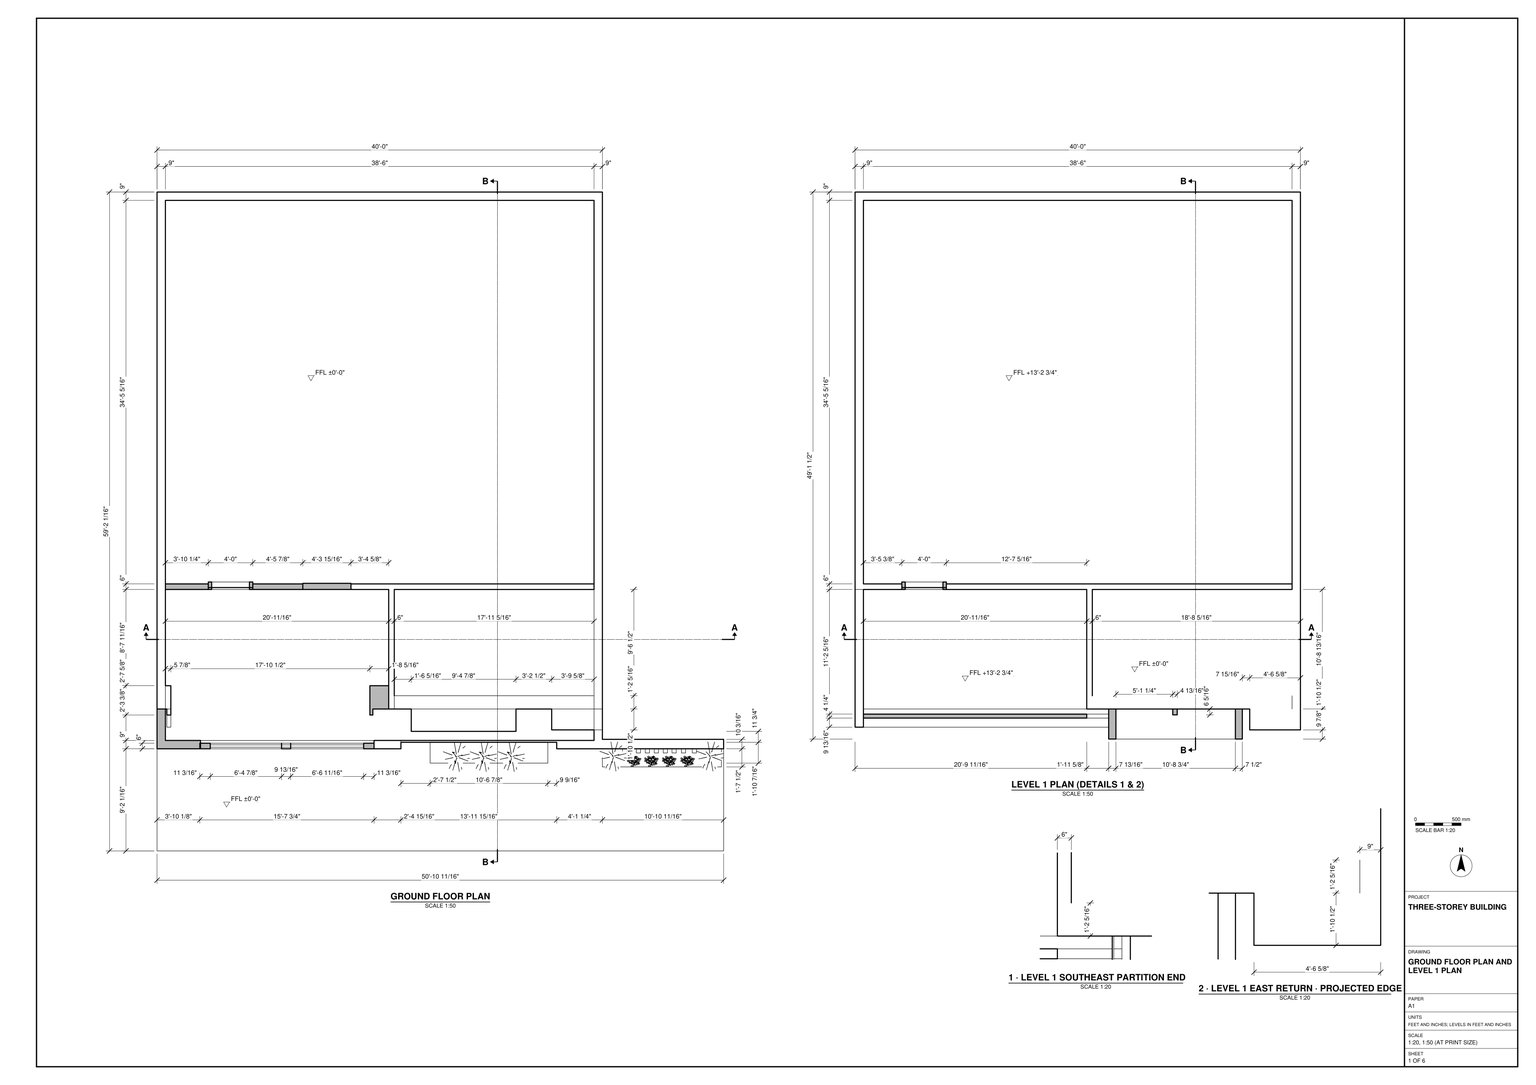
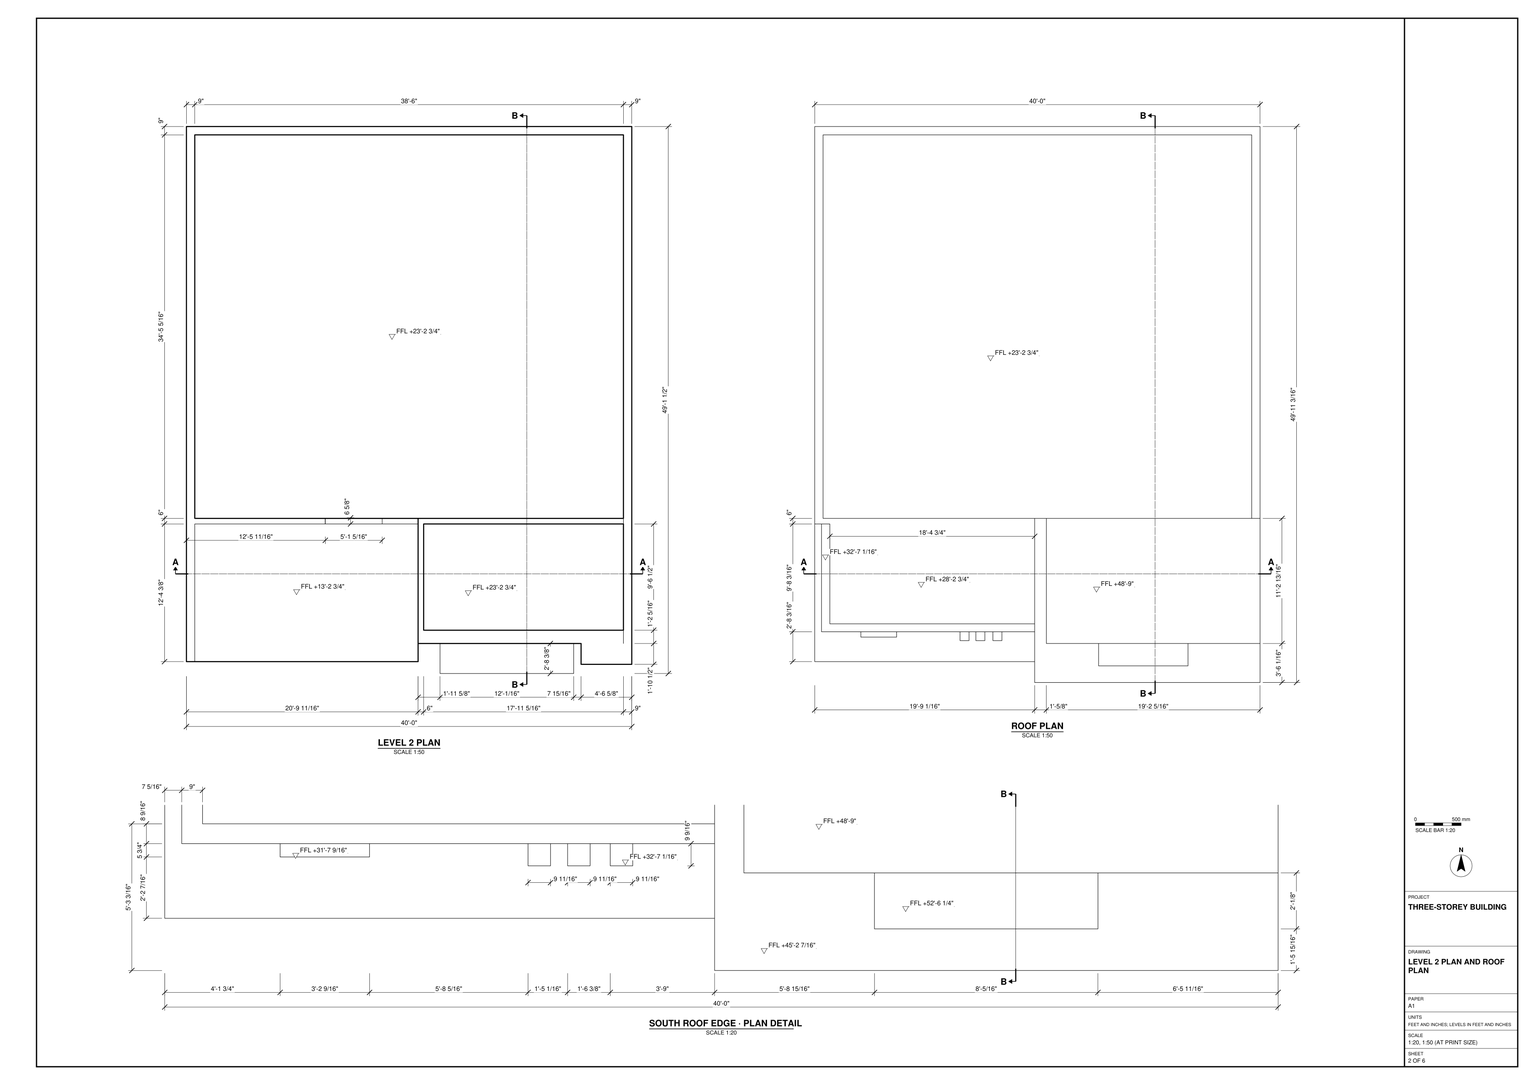
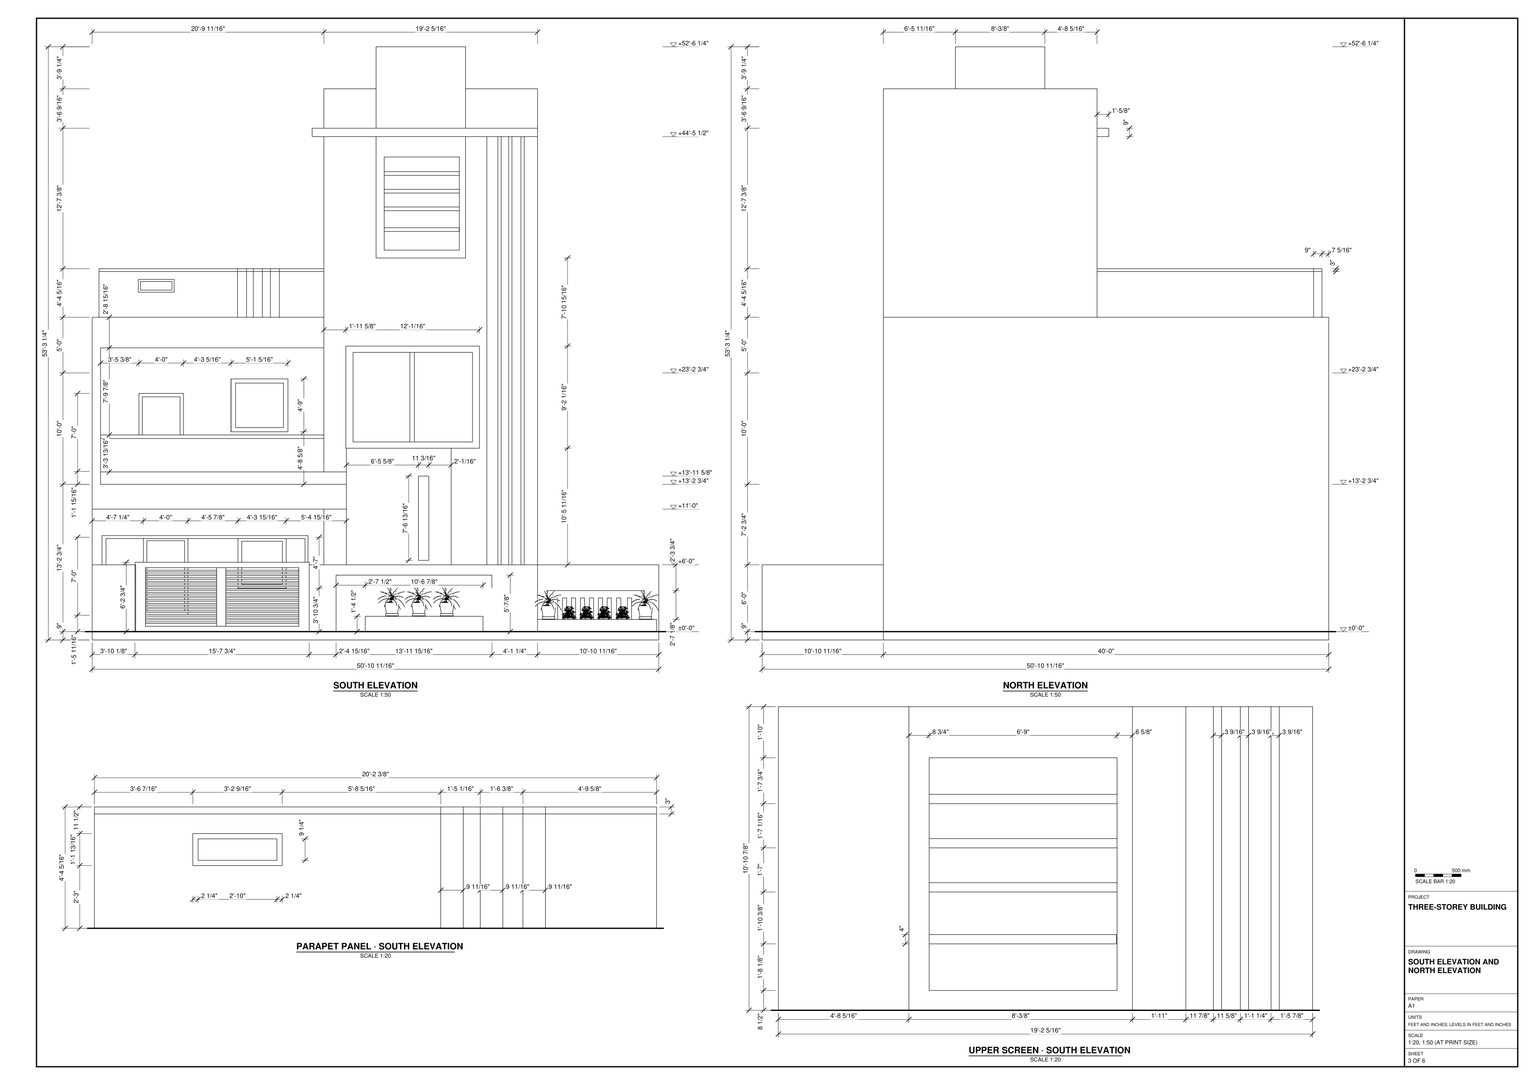
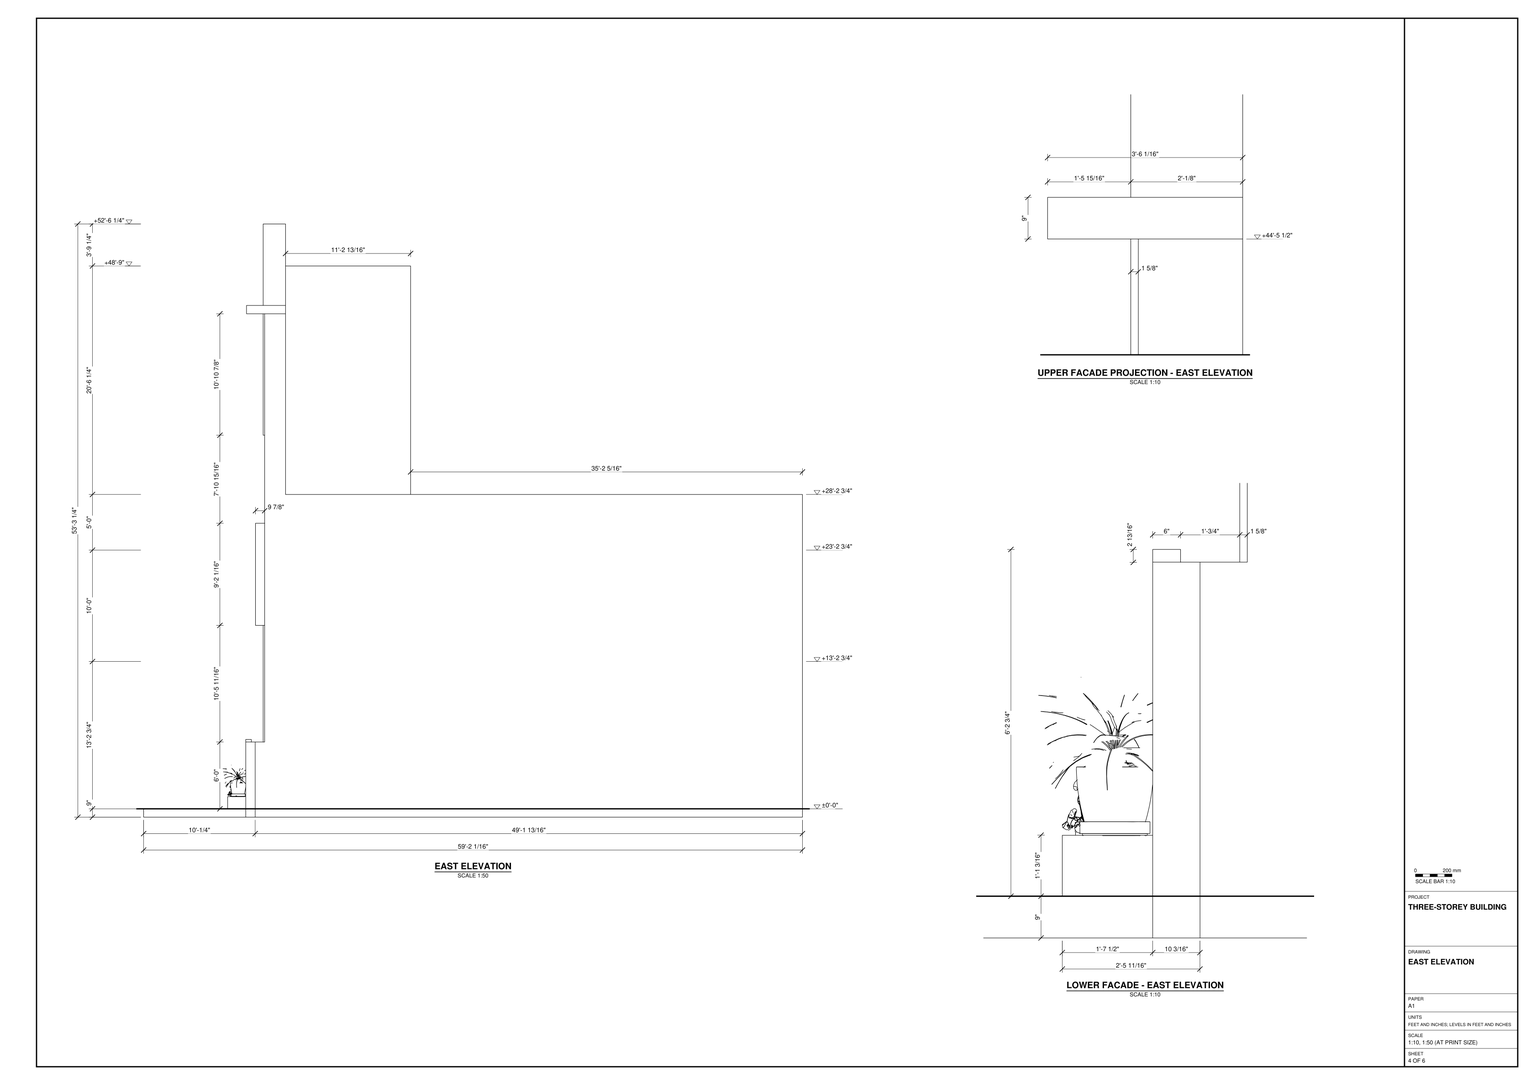
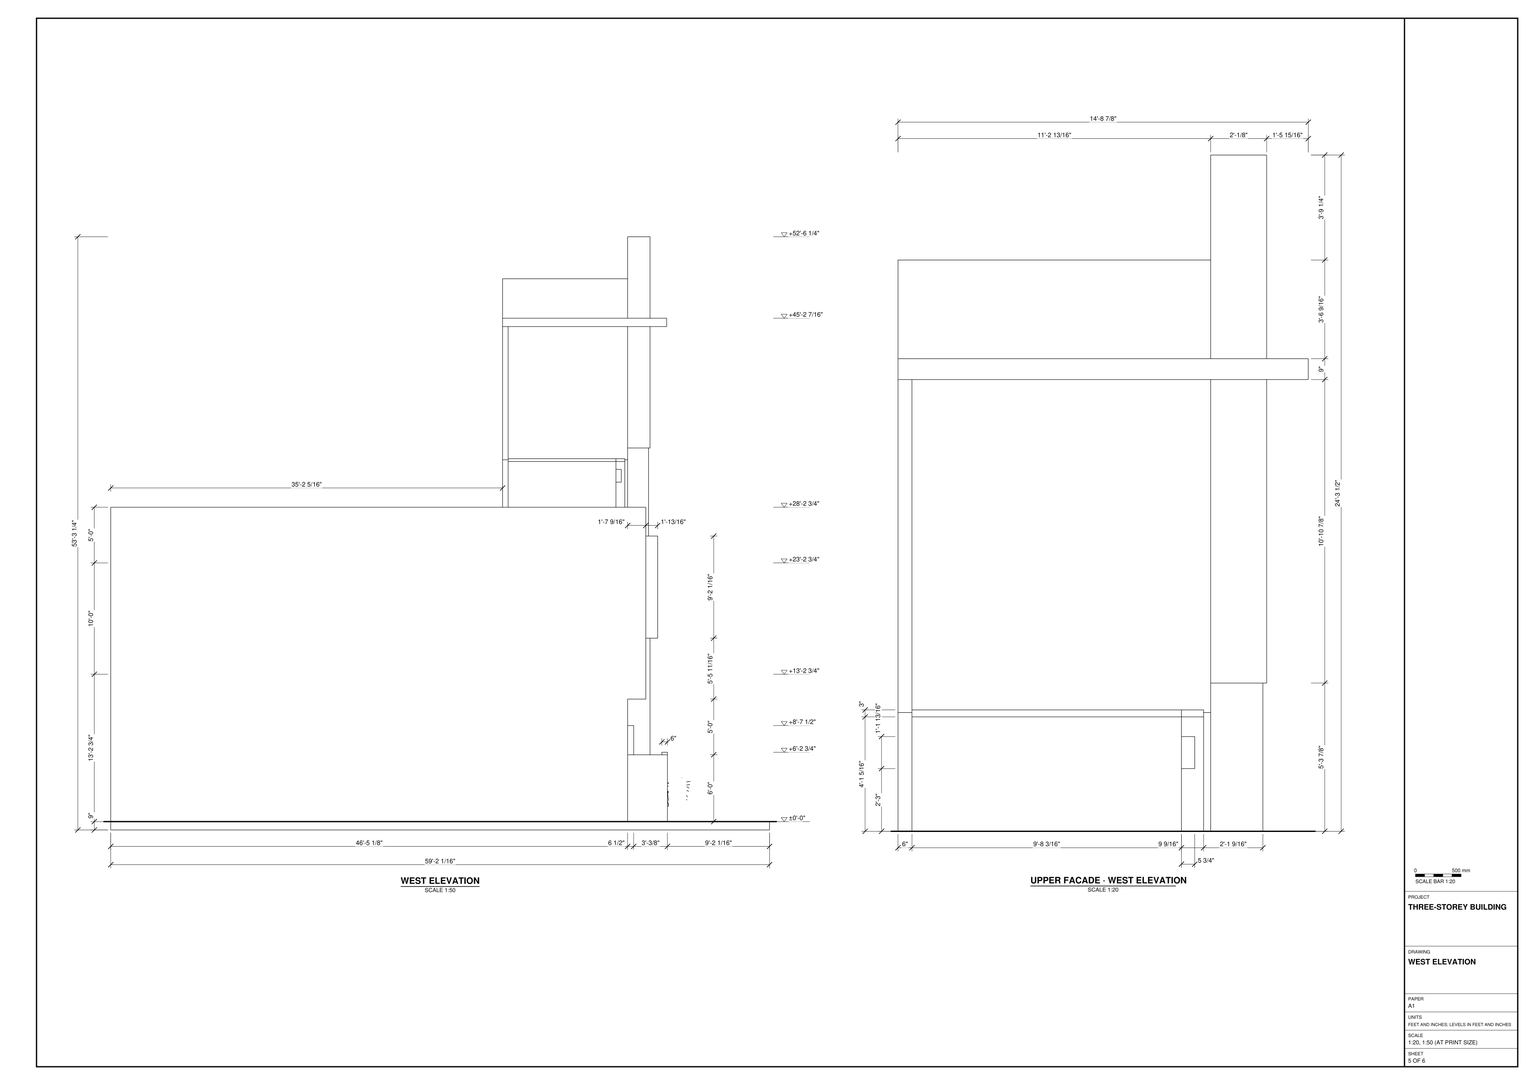
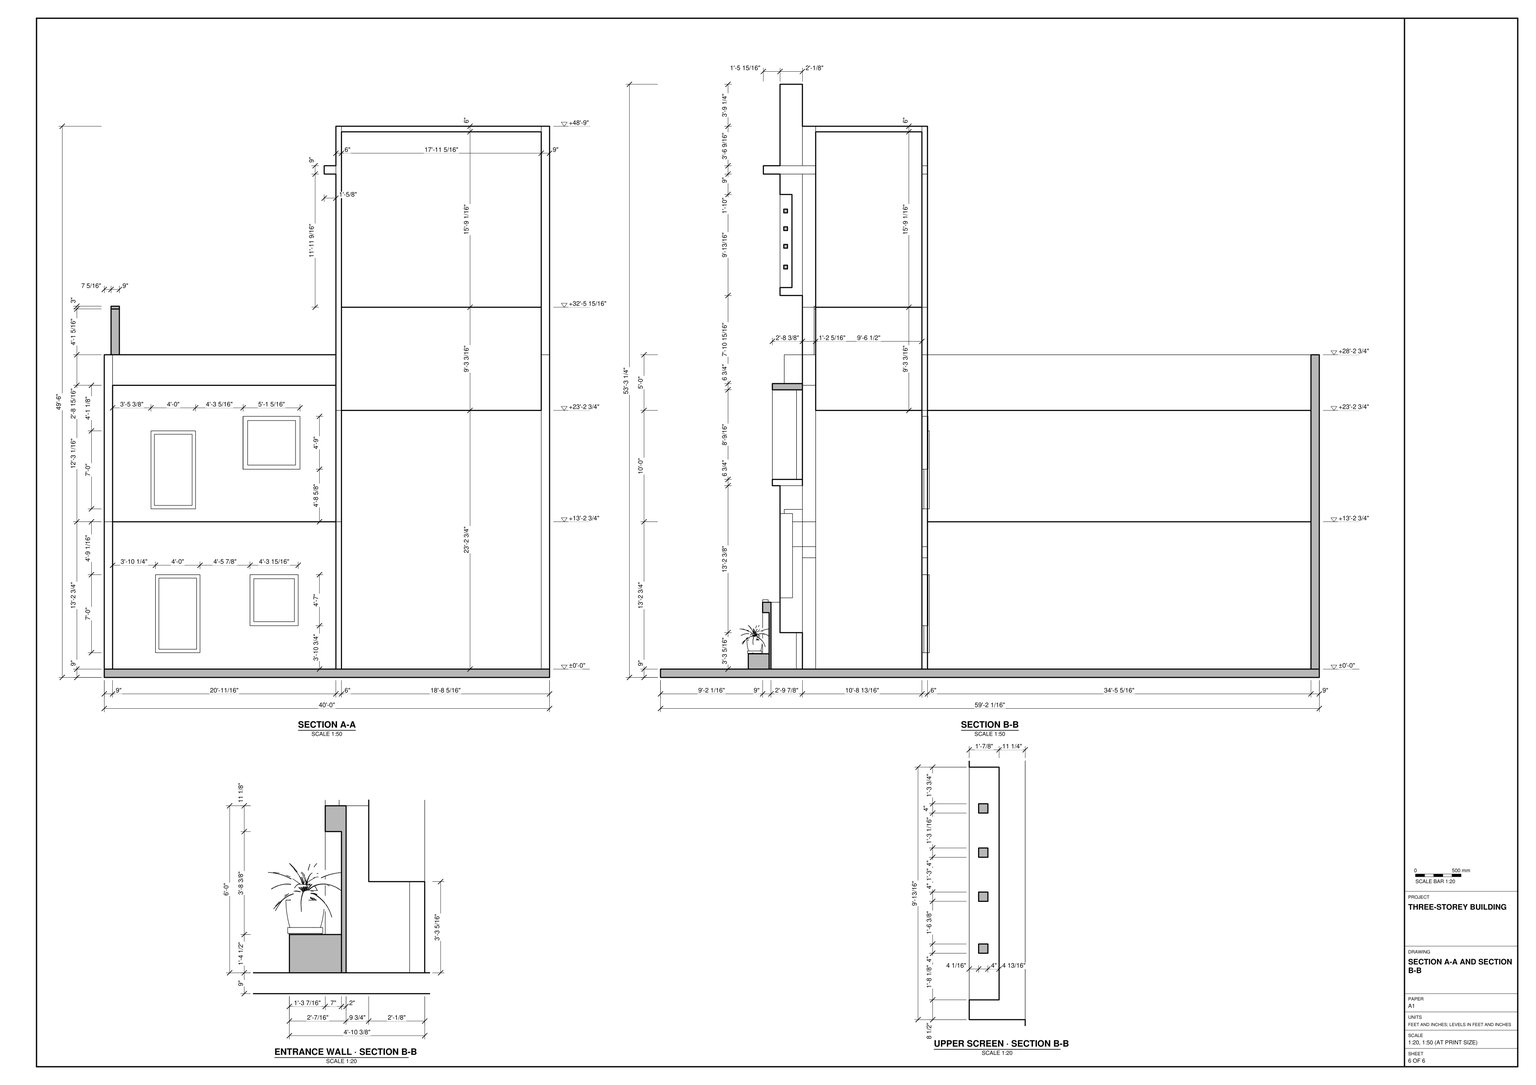
Build the three-storey building in SketchUp from task_files/diagram_01.pdf. Work in feet and inches. Including the front boundary and planters, the model shall measure 50'-10 11/16" along X, 59'-2 1/16" along Y and 53'-3 1/4" along Z. Set the finished floor levels to ±0'-0", +13'-2 3/4" and +23'-2 3/4".

Lay out the 40'-0" wide main block with a large undivided rear space and two unequal front bays. Follow the drawn wall thicknesses and opening positions. Use the floor level marked in each bay to determine where each slab stops rather than extending every slab across the whole footprint. Model the floor and roof slabs, parapets and projecting edges. Include stairs, built-in joinery and main furniture only where shown.

On the south elevation, distinguish the lower recessed bay from the tall bay with its framed opening, banded upper screen and vertical fins. Carry the stepped roof profile around to the plain north elevation. Model the slatted gate and the planted areas along the south boundary. Decor and loose items, including plants, may be any suitable library components.

Keep shell elements such as walls, slabs and roofs, and each furniture or joinery piece, in separate groups or components. Use components for repeated parts. Save one SketchUp model as output_files/three_storey_building_with_a_stepped_south_facade.skp.

# SketchUp Ruby script. Lengths in inches.
U = 1.inch
M = Sketchup.active_model
def pt(a) = Geom::Point3d.new(a.map { |v| v * U })
def face(e, loops, mat)
  f = e.add_face(loops[0].map { |a| pt(a) })
  loops[1..].each { |l| e.add_face(l.map { |a| pt(a) }).erase! }
  f.material = f.back_material = mat if mat
  f
end
# faces: each face lists its corners as indices into pts; further lists are holes
def faces(e, pts, list, mat = nil) = list.each { |f| face(e, (f[0].is_a?(Array) ? f : [f]).map { |l| l.map { |i| pts[i] } }, mat) }
# xy, xz, yz: faces in a plane at the given z, y or x. An outline is a flat list of corners, or four numbers for a rectangle; further outlines are holes
def ring(l) = l.size == 4 ? [[l[0], l[1]], [l[2], l[1]], [l[2], l[3]], [l[0], l[3]]] : l.each_slice(2).to_a
def flat(e, list, mat, &to3) = list.each { |f| face(e, (f[0].is_a?(Array) ? f : [f]).map { |l| ring(l).map { |u, v| to3.(u, v) } }, mat) }
def xy(e, z, list, mat = nil) = flat(e, list, mat) { |x, y| [x, y, z] }
def xz(e, y, list, mat = nil) = flat(e, list, mat) { |x, z| [x, y, z] }
def yz(e, x, list, mat = nil) = flat(e, list, mat) { |y, z| [x, y, z] }
def lines(e, pts, list) = list.each { |a, b| e.add_line(pt(pts[a]), pt(pts[b])) }
# prism: a flat outline (further loops are holes) pulled along v
def prism(e, loops, v, mat = nil)
  f = face(e, loops, mat); d = Geom::Vector3d.new(v.map { |x| x * U })
  f.pushpull(f.normal.samedirection?(d) ? d.length : -d.length)
end
def box(e, o, s, mat = nil) = prism(e, [[o, [o[0] + s[0], o[1], o[2]], [o[0] + s[0], o[1] + s[1], o[2]], [o[0], o[1] + s[1], o[2]]]], [0, 0, s[2]], mat)
def at(x, y, z, deg = 0) = Geom::Transformation.translation(pt([x, y, z])) * Geom::Transformation.rotation(ORIGIN, Z_AXIS, deg.degrees)
def axes(o, x, y, z) = Geom::Transformation.new([*x, 0, *y, 0, *z, 0, *pt(o).to_a, 1])
def part(name) = M.definitions.add(name)
# library, detail: a bought-in or finely detailed component or shape, given as its bounding box
def library(name, o, s) = part(name).tap { |d| box(d.entities, o, s) }
def detail(e, o, s) = box(e.add_group.entities, o, s)
def put(e, d, t, mat = nil) = e.add_instance(d, t).tap { |i| i.material = mat if mat }
def group(e, t, mat = nil) = e.add_group.tap { |g| g.transformation = t; g.material = mat if mat }.entities
root = M.entities
M.materials.add("LOTUS_leaf1").color = [82, 108, 38]
M.materials.add("Paint Cast Metal Grey1").color = [102, 98, 98]
M.materials.add("[Blacktop Old 01]").color = [132, 136, 139]
M.materials.add("[Color A08]").color = [69, 0, 0]
M.materials.add("[Color A08]1").color = [56, 0, 0]
M.materials.add("[Color A08]2").color = [71, 0, 0]
M.materials.add("[Color C01]").color = [255, 229, 204]
M.materials.add("[Color E01]").color = [255, 255, 204]
M.materials.add("[Color H08]").color = [78, 102, 102]
M.materials.add("[Color I04]").color = [22, 97, 255]
M.materials.add("[Color K01]").color = [255, 204, 255]
M.materials.add("[Color L03]").color = [255, 101, 178]
M.materials.add("[Color M00]").color = [255, 255, 255]
M.materials.add("[Color M02]").color = [198, 198, 198]
M.materials.add("[Color M05]").color = [114, 114, 114]
M.materials.add("[Color M08]").color = [30, 30, 30]
M.materials.add("[Concrete Block Retaining Gray]").color = [121, 121, 121]
M.materials.add("[Grass Dark Green]").color = [106, 157, 55]
M.materials.add("[Groundcover Rock Crushed Multi]").color = [143, 133, 129]
M.materials.add("[Metal Silver]").color = [234, 233, 238]
M.materials.add("[Pavers with Grass Brick]").color = [187, 192, 176]
M.materials.add("[Stone Vein Gray]").color = [166, 165, 165]
M.materials.add("[Translucent Glass Gray]").color = [128, 128, 128]
M.materials["[Translucent Glass Gray]"].alpha = 0.5
M.materials.add("[Translucent Glass Sky Reflection]").color = [126, 138, 183]
M.materials["[Translucent Glass Sky Reflection]"].alpha = 0.52
M.materials.add("[Windmill]").color = [39, 99, 236]
M.materials.add("[Windmill]1").color = [50, 82, 236]
M.materials.add("[Wood Fence]").color = [142, 67, 30]
M.materials.add("[Wood Floor Parquet]").color = [145, 89, 39]
M.materials.add("[Wood Lumber ButtJoined]").color = [164, 152, 112]
M.materials.add("bud1").color = [150, 156, 130]
M.materials.add("grit1").color = [185, 175, 150]
M.materials.add("steam_lotus1").color = [54, 65, 20]
c1 = part("Gruppe\#59")
xz(c1.entities,0,[[0,0,19.69,47.24]])
c2 = part("Gruppe\#58")
xz(c2.entities,0,[[0,0,19.69,47.24]])
c3 = part("buchsbaum")
xy(c3.entities,8.86,[[9.1875,3.27,15.1,9.1875,9.1875,15.1,3.27,9.1875]])
p = [[9.1875,4.45,0],[9.1875,3.27,8.86],[3.27,9.1875,8.86],[4.45,9.1875,0],[13.92,9.1875,0],[15.1,9.1875,8.86],
  [9.1875,15.1,8.86],[9.1875,13.92,0]]
faces(c3.entities,p,[[0,1,2,3],[4,5,1,0],[3,2,6,7],[7,6,5,4]])
put(c3.entities,c1,at(0,9.84,0))
put(c3.entities,c2,at(9.84,0,0,90))
c4 = library("plants",[-16.3,-15.81,0],[32.6,31.62,37.8])
c5 = library("Group\#8",[-142.52,-120.11,41.88],[289.73,289.12,19.34])
c6 = library("Group\#10",[-178.09,-198.15,32.25],[355.38,385.92,255.57])
c7 = library("Group\#6",[-158.6,-197.39,34.74],[309.58,325.03,250.96])
c8 = library("Group\#7",[-148.5625,-125.53,0.71],[301.67,301.67,62.99])
c9 = library("Group\#9",[-215.02,-238.32,10.29],[429.97,469.64,305.33])
c10 = part("Potted plant")
p = [[215.02,238.32,0],[216.02,238.32,0],[216.02,239.32,0]]
lines(c10.entities,p,[[0,1],[1,2],[2,0]])
put(c10.entities,c5,at(215.02,238.32,0),"grit1")
put(c10.entities,c6,at(215.02,238.32,0),"steam_lotus1")
put(c10.entities,c7,at(215.02,238.32,0),"bud1")
put(c10.entities,c8,at(215.02,238.32,0),"Paint Cast Metal Grey1")
put(c10.entities,c9,at(215.02,238.32,0),"LOTUS_leaf1")
c11 = part("Group\#1")
xy(c11.entities,0,[[0,0,48,2.0625],[0,2.0625,48,8.0625]],"[Color A08]")
xy(c11.entities,3.66,[[3.66,0,44.34,2.0625]])
xy(c11.entities,3.66,[[3.66,2.0625,44.34,8.0625]],"[Color A08]")
xy(c11.entities,80.34,[[3.66,0,44.34,2.0625]])
xy(c11.entities,80.34,[[3.66,2.0625,44.34,8.0625]],"[Color A08]")
xy(c11.entities,84,[[0,0,48,2.0625],[0,2.0625,48,8.0625]],"[Color A08]")
xz(c11.entities,0,[[[0,0,48,84],[3.66,3.66,44.34,80.34]]],"[Color A08]")
xz(c11.entities,2.0625,[[[0,0,48,84],[3.66,3.66,44.34,80.34]]])
xz(c11.entities,2.0625,[[3.66,3.66,44.34,80.34]],"[Translucent Glass Gray]")
xz(c11.entities,8.0625,[[[0,0,48,84],[3.66,3.66,44.34,80.34]]],"[Color A08]")
yz(c11.entities,0,[[0,0,2.0625,84],[2.0625,0,8.0625,84]],"[Color A08]")
yz(c11.entities,3.66,[[0,3.66,2.0625,80.34]])
yz(c11.entities,3.66,[[2.0625,3.66,8.0625,80.34]],"[Color A08]")
yz(c11.entities,44.34,[[0,3.66,2.0625,80.34]])
yz(c11.entities,44.34,[[2.0625,3.66,8.0625,80.34]],"[Color A08]")
yz(c11.entities,48,[[0,0,2.0625,84],[2.0625,0,8.0625,84]],"[Color A08]")
c12 = part("Group\#2")
xy(c12.entities,0,[[0,0,48.5,6.625]],"[Color A08]1")
xy(c12.entities,3.83,[[3.83,0,44.67,6.625]],"[Color A08]1")
xy(c12.entities,44.67,[[3.83,0,44.67,6.625]],"[Color A08]1")
xy(c12.entities,48.5,[[0,0,48.5,6.625]],"[Color A08]1")
xz(c12.entities,0,[[[0,0,48.5,48.5],[3.83,3.83,44.67,44.67]]],"[Color A08]1")
xz(c12.entities,0,[[3.83,3.83,44.67,44.67]],"[Translucent Glass Gray]")
xz(c12.entities,6.625,[[[0,0,48.5,48.5],[3.83,3.83,44.67,44.67]]],"[Color A08]1")
yz(c12.entities,0,[[0,0,6.625,48.5]],"[Color A08]1")
yz(c12.entities,3.83,[[0,3.83,6.625,44.67]],"[Color A08]1")
yz(c12.entities,44.67,[[0,3.83,6.625,44.67]],"[Color A08]1")
yz(c12.entities,48.5,[[0,0,6.625,48.5]],"[Color A08]1")
c13 = library("Group\#3",[0,0,0],[143.3125,6,110.5])
xy(root,0,[[0,0,0,710.0625,480,710.0625,480,120.25,610.6875,120.25,610.6875,0]])
xy(root,9,[[0,110.0625,0,152.94,9,152.94,9,119.0625,46.86,119.0625,46.86,110.0625],[233.89,110.0625,262.84,119.0625],[430.78,110.0625,430.78,117.0625,262.84,117.0625,262.84,119.0625,471,119.0625,471,130.44,480,130.44,480,120.25,610.6875,120.25,610.6875,110.0625],[425.36,130.44,471,152.94],[471,130.44,480,152.94],
  [10.59,133.375,14.875,146.4375],[10.59,146.4375,14.875,152.94],[0,152.94,0,710.0625,480,710.0625,480,152.94,471,152.94,471,701.0625,9,701.0625,9,152.94],[249.6875,152.94,249.6875,281.75,9,281.75,9,287.75,471,287.75,471,281.75,255.6875,281.75,255.6875,152.94],[9,152.94,14.875,178.07],
  [229.4,152.94,249.6875,178.07],[255.6875,152.94,471,167.25],[255.6875,167.25,471,281.75],[9,287.75,471,701.0625]])
xy(root,9,[[0,0,610.6875,0,610.6875,110.0625,608.3125,110.0625,608.3125,90.5625,480,90.5625,480,110.0625,430.78,110.0625,430.78,117.0625,421.21,117.0625,421.21,94.625,294.33,94.625,294.33,117.0625,262.84,117.0625,262.84,110.0625,233.89,110.0625,233.89,119.0625,46.86,119.0625,46.86,110.0625,0,110.0625],[294.33,94.625,421.21,117.0625]],"[Pavers with Grass Brick]")
xy(root,9,[[9,119.0625,471,119.0625,471,130.44,425.36,130.44,425.36,152.94,232.59,152.94,232.59,146.4375,229.4,146.4375,229.4,178.07,249.6875,178.07,249.6875,281.75,9,281.75,9,178.07,14.875,178.07,14.875,133.375,10.59,133.375,10.59,152.94,9,152.94]],"[Stone Vein Gray]")
xy(root,22.125,[[497.15,105.5625,501.67,110.0625],[506.84,105.5625,511.36,110.0625],[516.52,105.5625,521.04,110.0625],[526.21,105.5625,530.73,110.0625],[535.9,105.5625,540.42,110.0625],
  [545.59,105.5625,550.11,110.0625],[555.02,105.5625,559.54,110.0625],[565.21,105.5625,569.73,110.0625],[576.84,105.5625,581.36,110.0625]],"[Color M00]")
xy(root,22.125,[[480,90.5625,608.3125,90.5625,608.3125,110.0625,581.36,110.0625,581.36,105.5625,576.84,105.5625,576.84,110.0625,569.73,110.0625,569.73,105.5625,565.21,105.5625,565.21,110.0625,559.54,110.0625,559.54,105.5625,555.02,105.5625,555.02,110.0625,550.11,110.0625,550.11,105.5625,545.59,105.5625,545.59,110.0625,540.42,110.0625,540.42,105.5625,535.9,105.5625,535.9,110.0625,530.73,110.0625,530.73,105.5625,526.21,105.5625,526.21,110.0625,521.04,110.0625,521.04,105.5625,516.52,105.5625,516.52,110.0625,511.36,110.0625,511.36,105.5625,506.84,105.5625,506.84,110.0625,501.67,110.0625,501.67,105.5625,497.15,105.5625,497.15,110.0625,480,110.0625]],"[Groundcover Rock Crushed Multi]")
xy(root,25.5,[[294.33,94.625,421.21,117.0625]],"[Grass Dark Green]")
xy(root,26.7,[[55.22,281.75,103.22,287.75]])
xy(root,45.24,[[497.15,105.5625,501.67,110.0625],[506.84,105.5625,511.36,110.0625],[516.52,105.5625,521.04,110.0625],[526.21,105.5625,530.73,110.0625],[535.9,105.5625,540.42,110.0625],
  [545.59,105.5625,550.11,110.0625],[555.02,105.5625,559.54,110.0625],[565.21,105.5625,569.73,110.0625],[576.84,105.5625,581.36,110.0625]],"[Color M00]")
xy(root,48.3,[[274,128.82,386.875,152.94]])
xy(root,55.75,[[157.1,281.75,209.04,287.75]])
xy(root,69.875,[[262.84,110.0625,430.78,117.0625]])
xy(root,81,[[0,110.0625,46.86,110.0625,46.86,119.0625,9,119.0625,9,152.94,0,152.94],[233.89,110.0625,480,110.0625,480,130.44,471,130.44,471,119.0625,233.89,119.0625],[480,110.0625,610.6875,120.25]])
xy(root,85.8,[[351.63,128.82,362.82,142.32]])
xy(root,109.25,[[14.875,146.4375,229.4,152.94],[14.875,152.94,229.4,178.07]])
xy(root,110.7,[[55.22,281.75,103.22,287.75]])
xy(root,110.75,[[157.1,281.75,209.04,287.75]])
xy(root,112.5,[[10.59,146.4375,232.59,152.94]])
xy(root,141,[[0,133.375,277.5,152.94],[9,152.94,249.6875,178.07]])
xy(root,167.75,[[9,133.375,277.5,152.94],[9,287.75,471,701.0625]])
xy(root,167.75,[[9,152.94,249.6875,281.75]],"[Stone Vein Gray]")
xy(root,176.61,[[351.63,128.82,362.82,142.32]])
xy(root,181.125,[[9,133.375,277.5,143.16],[9,143.16,249.6875,147.43],[249.6875,143.16,277.5,147.43],[9,147.43,277.5,152.94]])
xy(root,181.71,[[50.39,281.75,98.39,287.75]])
xy(root,206.66,[[273.34,120.57,273.34,152.94,274,152.94,274,128.82,386.875,128.82,386.875,152.94,417.39,152.94,417.39,120.57]])
xy(root,213.4,[[281.15,120.57,409.9,120.57,409.9,152.94,347.2,152.94,347.2,146.63,342.39,146.63,342.39,152.94,281.15,152.94],[342.39,146.63,347.2,152.94]])
xy(root,217.125,[[9,143.16,249.6875,147.43]])
xy(root,220.9375,[[9,143.16,249.6875,147.43]],"[Metal Silver]")
xy(root,224.35,[[149.55,281.75,210.98,287.75]])
xy(root,265.71,[[50.39,281.75,98.39,287.75]])
xy(root,281.35,[[149.55,281.75,210.98,287.75]])
xy(root,287.75,[[255.6875,167.25,471,281.75]])
xy(root,287.75,[[9,287.75,471,701.0625]],"[Blacktop Old 01]")
xy(root,309.96,[[281.15,120.57,281.15,152.94,342.39,152.94,342.39,146.63,347.2,146.63,347.2,152.94,409.9,152.94,409.9,120.57],[342.39,146.63,347.2,152.94]])
xy(root,314.81,[[9,133.375,249.6875,281.75]])
xy(root,316.71,[[273.34,120.57,417.39,152.94]])
xy(root,347.75,[[0,133.375,249.6875,133.375,249.6875,165.57,201.77,165.57,201.77,156,192.06,156,192.06,165.57,183.39,165.57,183.39,156,173.69,156,173.69,165.57,166.33,165.57,166.33,156,156.62,156,156.62,165.57,7.33,165.57,7.33,281.75,0,281.75],[156.62,156,156.62,165.57,7.33,165.57,7.33,281.75,16.3,281.75,16.3,174.11,249.6875,174.11,249.6875,165.57,201.77,165.57,201.77,156,192.06,156,192.06,165.57,183.39,165.57,183.39,156,173.69,156,173.69,165.57,166.33,165.57,166.33,156],[16.3,174.11,249.6875,174.11,249.6875,287.75,9,287.75,9,701.0625,471,701.0625,471,287.75,480,287.75,480,710.0625,0,710.0625,0,281.75,16.3,281.75]])
xy(root,374.77,[[49.74,159.82,88.29,165.57]])
xy(root,377.05,[[52.02,159.82,86.02,165.57]])
xy(root,386.3,[[52.02,159.82,86.02,165.57]])
xy(root,388.57,[[49.74,159.82,88.29,165.57]])
xy(root,397.0625,[[156.62,156,166.33,165.57],[173.69,156,183.39,165.57],[192.06,156,201.77,165.57],[7.33,165.57,7.33,281.75,16.3,281.75,16.3,174.11,249.6875,174.11,249.6875,165.57]])
xy(root,398.9375,[[255.6875,167.25,471,281.6875]])
xy(root,400.0625,[[156.62,156,166.33,165.57],[7.33,165.57,249.6875,165.57,249.6875,174.11,16.3,174.11,16.3,281.75,7.33,281.75]])
xy(root,400.0625,[[173.69,156,183.39,165.57],[192.06,156,201.77,165.57]],"[Color M02]")
xy(root,411.63,[[305.97,128.82,402.34,152.94]],"[Color L03]")
xy(root,420.16,[[314.71,128.82,395.71,141.69]],"[Color L03]")
xy(root,440.26,[[314.71,132.87,395.46,136.87]],"[Color A08]2")
xy(root,444.26,[[314.71,132.87,395.46,136.87]],"[Color A08]2")
xy(root,462.63,[[314.71,132.87,396.08,136.87]],"[Color A08]2")
xy(root,466.63,[[314.71,132.87,396.08,136.87]],"[Color A08]2")
xy(root,481.63,[[314.71,132.87,395.71,136.87]],"[Color A08]2")
xy(root,485.63,[[314.71,132.87,395.71,136.87]],"[Color A08]2")
xy(root,500.69,[[314.71,132.87,396.33,136.87]],"[Color A08]2")
xy(root,504.69,[[314.71,132.87,396.33,136.87]],"[Color A08]2")
xy(root,520.47,[[314.71,128.82,395.71,141.69]],"[Color L03]")
xy(root,542.48,[[237.0625,110.88,237.0625,281.75,249.6875,281.75,249.6875,152.94,305.97,152.94,305.97,128.82,402.34,128.82,402.34,152.94,425.36,152.94,425.36,130.44,480,130.44,480,110.88],[425.36,130.44,480,152.94],[237.0625,281.75,249.6875,287.75]])
xy(root,551.46,[[237.0625,110.88,480,110.88,480,152.94,402.34,152.94,402.34,128.82,305.97,128.82,305.97,152.94,249.6875,152.94,249.6875,287.75,237.0625,287.75]])
xy(root,588,[[255.6875,167.25,471,281.75]])
xy(root,594,[[249.6875,152.94,480,287.75]],"[Windmill]")
xy(root,639.25,[[305.97,128.82,402.34,152.94]],"[Color L03]")
xz(root,0,[[0,0,610.6875,9]],"[Color M08]")
xz(root,90.5625,[[480,9,608.3125,22.125]],"[Concrete Block Retaining Gray]")
xz(root,94.625,[[294.33,9,421.21,25.5]],"[Concrete Block Retaining Gray]")
xz(root,105.5625,[[497.15,22.125,501.67,45.24],[506.84,22.125,511.36,45.24],[516.52,22.125,521.04,45.24],[526.21,22.125,530.73,45.24],[535.9,22.125,540.42,45.24],
  [545.59,22.125,550.11,45.24],[555.02,22.125,559.54,45.24],[565.21,22.125,569.73,45.24],[576.84,22.125,581.36,45.24]],"[Color M00]")
xz(root,110.0625,[[0,9,46.86,81],[233.89,9,262.84,9,262.84,69.875,430.78,69.875,430.78,9,480,9,480,81,233.89,81]])
xz(root,110.0625,[[480,9,490.32,22.125],[490.32,9,595,22.125],[595,9,608.3125,22.125]],"[Pavers with Grass Brick]")
xz(root,110.0625,[[608.3125,9,610.6875,9,610.6875,81,480,81,480,22.125,490.32,22.125,490.32,53.25,595,53.25,595,22.125,608.3125,22.125]],"[Wood Floor Parquet]")
xz(root,110.0625,[[490.32,22.125,497.15,22.125,497.15,45.24,501.67,45.24,501.67,22.125,506.84,22.125,506.84,45.24,511.36,45.24,511.36,22.125,516.52,22.125,516.52,45.24,521.04,45.24,521.04,22.125,526.21,22.125,526.21,45.24,530.73,45.24,530.73,22.125,535.9,22.125,535.9,45.24,540.42,45.24,540.42,22.125,545.59,22.125,545.59,45.24,550.11,45.24,550.11,22.125,555.02,22.125,555.02,45.24,559.54,45.24,559.54,22.125,565.21,22.125,565.21,45.24,569.73,45.24,569.73,22.125,576.84,22.125,576.84,45.24,581.36,45.24,581.36,22.125,595,22.125,595,53.25,490.32,53.25]],"[Wood Lumber ButtJoined]")
xz(root,110.88,[[237.0625,542.48,480,551.46]])
xz(root,117.0625,[[294.33,9,421.21,25.5]],"[Pavers with Grass Brick]")
xz(root,117.0625,[[262.84,9,294.33,9,294.33,25.5,421.21,25.5,421.21,9,430.78,9,430.78,69.875,262.84,69.875]],"[Wood Fence]")
xz(root,119.0625,[[9,9,46.86,81],[233.89,9,262.84,81],[262.84,9,471,81]])
xz(root,120.25,[[480,9,610.6875,81]],"[Color K01]")
xz(root,120.25,[[480,0,610.6875,9]],"[Color M08]")
xz(root,120.57,[[[273.34,206.66,417.39,316.71],[281.15,213.4,409.9,309.96]]])
xz(root,128.82,[[[274,48.3,386.875,206.66],[351.63,85.8,362.82,176.61]],[[305.97,411.63,402.34,542.48],[314.71,420.16,395.71,520.47]],[305.97,551.46,402.34,639.25]],"[Color L03]")
xz(root,130.44,[[437.22,9,440.78,542.48],[448.85,9,452.4,542.48],[462.1,9,465.65,542.48]])
xz(root,130.44,[[425.36,9,437.22,542.48],[440.78,9,448.85,542.48],[452.4,9,462.1,542.48],[465.65,9,471,9,471,81,480,81,480,542.48,465.65,542.48]],"[Color H08]")
xz(root,132.87,[[314.71,440.26,395.46,444.26],[314.71,462.63,396.08,466.63],[314.71,481.63,395.71,485.63],[314.71,500.69,396.33,504.69]],"[Color A08]2")
xz(root,133.375,[[0,141,277.5,141,277.5,167.75,9,167.75,9,314.81,249.6875,314.81,249.6875,347.75,0,347.75]])
xz(root,133.375,[[9,167.75,277.5,181.125]],"[Wood Fence]")
xz(root,136.87,[[314.71,440.26,395.46,444.26]])
xz(root,136.87,[[314.71,462.63,396.08,466.63],[314.71,481.63,395.71,485.63],[314.71,500.69,396.33,504.69]],"[Color A08]2")
xz(root,141.69,[[314.71,420.16,395.71,520.47]],"[Translucent Glass Sky Reflection]")
xz(root,142.32,[[351.63,85.8,362.82,176.61]])
xz(root,143.16,[[9,217.125,249.6875,220.9375]],"[Metal Silver]")
xz(root,143.16,[[9,181.125,249.6875,217.125]],"[Translucent Glass Gray]")
xz(root,146.4375,[[10.59,9,14.875,9,14.875,109.25,229.4,109.25,229.4,9,232.59,9,232.59,112.5,10.59,112.5]])
xz(root,146.63,[[342.39,213.4,347.2,309.96]])
xz(root,147.43,[[9,217.125,249.6875,220.9375]],"[Metal Silver]")
xz(root,147.43,[[9,181.125,249.6875,217.125]],"[Translucent Glass Gray]")
xz(root,152.94,[[0,9,9,81],[9,141,249.6875,167.75],[249.6875,141,274,167.75],[274,141,277.5,167.75],[9,167.75,249.6875,181.125],
  [249.6875,167.75,274,181.125],[274,167.75,277.5,181.125],[[273.34,206.66,417.39,316.71],[281.15,213.4,409.9,309.96]],[342.39,213.4,347.2,309.96]])
xz(root,152.94,[[9,9,10.59,9,10.59,112.5,232.59,112.5,232.59,9,249.6875,9,249.6875,141,0,141,0,81,9,81]],"[Color I04]")
xz(root,152.94,[[305.97,594,402.34,639.25]],"[Color L03]")
xz(root,152.94,[[281.15,213.4,342.39,309.96]],"[Translucent Glass Sky Reflection]")
xz(root,152.94,[[249.6875,9,425.36,9,425.36,542.48,402.34,542.48,402.34,411.63,305.97,411.63,305.97,542.48,249.6875,542.48,249.6875,181.125,274,181.125,274,206.66,273.34,206.66,273.34,316.71,417.39,316.71,417.39,206.66,386.875,206.66,386.875,48.3,274,48.3,274,141,249.6875,141],[249.6875,551.46,305.97,594],[402.34,551.46,480,594]],"[Windmill]")
xz(root,152.94,[[347.2,213.4,409.9,309.96]],"[Wood Fence]")
xz(root,156,[[156.62,397.0625,166.33,400.0625],[173.69,397.0625,183.39,400.0625],[192.06,397.0625,201.77,400.0625]],"[Color M02]")
xz(root,156,[[156.62,347.75,166.33,397.0625],[173.69,347.75,183.39,397.0625],[192.06,347.75,201.77,397.0625]],"[Color M05]")
xz(root,159.82,[[[49.74,374.77,88.29,388.57],[52.02,377.05,86.02,386.3]]])
xz(root,165.57,[[7.33,397.0625,156.62,400.0625],[156.62,397.0625,166.33,400.0625],[166.33,397.0625,173.69,400.0625],[173.69,397.0625,183.39,400.0625],[183.39,397.0625,192.06,400.0625],
  [192.06,397.0625,201.77,400.0625],[201.77,397.0625,249.6875,400.0625]])
xz(root,165.57,[[[7.33,347.75,156.62,397.0625],[49.74,374.77,88.29,388.57]],[166.33,347.75,173.69,397.0625],[183.39,347.75,192.06,397.0625],[201.77,347.75,249.6875,397.0625]],"[Color C01]")
xz(root,165.57,[[52.02,377.05,86.02,386.3]],"[Color M02]")
xz(root,167.25,[[255.6875,287.75,471,398.9375],[255.6875,398.9375,471,588]])
xz(root,174.11,[[16.3,347.75,249.6875,397.0625],[16.3,397.0625,249.6875,400.0625]])
xz(root,178.07,[[229.4,9,229.4,109.25,9,109.25,9,141,249.6875,141,249.6875,9],[9,9,14.875,109.25]])
xz(root,281.75,[[255.6875,9,471,287.75],[255.6875,287.75,471,398.9375],[7.33,347.75,16.3,397.0625],[7.33,397.0625,16.3,400.0625],[255.6875,398.9375,471,588]])
xz(root,281.75,[[[9,167.75,249.6875,314.81],[50.39,181.71,98.39,265.71],[149.55,224.35,210.98,281.35]]],"[Color C01]")
xz(root,281.75,[[[9,9,249.6875,167.75],[55.22,26.7,103.22,110.7],[157.1,55.75,209.04,110.75]]],"[Color E01]")
xz(root,287.75,[[[9,9,471,167.75],[55.22,26.7,103.22,110.7],[157.1,55.75,209.04,110.75]],[[9,167.75,471,287.75],[50.39,181.71,98.39,265.71],[149.55,224.35,210.98,281.35]],[9,287.75,249.6875,347.75]])
xz(root,287.75,[[249.6875,287.75,249.6875,594,480,594,480,347.75,471,347.75,471,287.75],[237.0625,542.48,249.6875,551.46]],"[Windmill]")
xz(root,701.0625,[[9,9,471,167.75],[9,167.75,471,287.75],[9,287.75,471,347.75]])
xz(root,710.0625,[[0,0,480,9]])
xz(root,710.0625,[[0,9,480,347.75]],"[Color K01]")
yz(root,0,[[110.0625,9,152.94,81]])
yz(root,0,[[152.94,9,152.94,141,133.375,141,133.375,347.75,710.0625,347.75,710.0625,9]],"[Color K01]")
yz(root,0,[[0,0,710.0625,9]],"[Color M08]")
yz(root,7.33,[[165.57,397.0625,281.75,400.0625]])
yz(root,7.33,[[165.57,347.75,281.75,397.0625]],"[Color C01]")
yz(root,9,[[119.0625,9,152.94,81],[281.75,9,287.75,129],[287.75,9,701.0625,167.75],[281.75,129,287.75,141],[152.94,141,281.75,167.75],
  [133.375,167.75,152.94,181.125],[287.75,167.75,701.0625,287.75],[143.16,181.125,147.43,217.125],[143.16,217.125,147.43,220.9375],[287.75,287.75,701.0625,347.75]])
yz(root,9,[[178.07,9,281.75,141],[152.94,167.75,281.75,167.75,281.75,314.81,133.375,314.81,133.375,181.125,143.16,181.125,143.16,220.9375,147.43,220.9375,147.43,181.125,152.94,181.125]],"[Color E01]")
yz(root,10.59,[[146.4375,9,152.94,112.5]])
yz(root,14.875,[[146.4375,9,178.07,109.25]],"[Color E01]")
yz(root,16.3,[[174.11,347.75,281.75,397.0625],[174.11,397.0625,281.75,400.0625]])
yz(root,46.86,[[110.0625,9,119.0625,81]])
yz(root,49.74,[[159.82,374.77,165.57,388.57]])
yz(root,50.39,[[281.75,181.71,287.75,265.71]])
yz(root,52.02,[[159.82,377.05,165.57,386.3]])
yz(root,55.22,[[281.75,26.7,287.75,110.7]])
yz(root,86.02,[[159.82,377.05,165.57,386.3]])
yz(root,88.29,[[159.82,374.77,165.57,388.57]])
yz(root,98.39,[[281.75,181.71,287.75,265.71]])
yz(root,103.22,[[281.75,26.7,287.75,110.7]])
yz(root,149.55,[[281.75,224.35,287.75,281.35]])
yz(root,156.62,[[156,397.0625,165.57,400.0625]],"[Color M02]")
yz(root,156.62,[[156,347.75,165.57,397.0625]],"[Color M05]")
yz(root,157.1,[[281.75,55.75,287.75,110.75]])
yz(root,166.33,[[156,397.0625,165.57,400.0625]],"[Color M02]")
yz(root,166.33,[[156,347.75,165.57,397.0625]],"[Color M05]")
yz(root,173.69,[[156,397.0625,165.57,400.0625]],"[Color M02]")
yz(root,173.69,[[156,347.75,165.57,397.0625]],"[Color M05]")
yz(root,183.39,[[156,397.0625,165.57,400.0625]],"[Color M02]")
yz(root,183.39,[[156,347.75,165.57,397.0625]],"[Color M05]")
yz(root,192.06,[[156,397.0625,165.57,400.0625]],"[Color M02]")
yz(root,192.06,[[156,347.75,165.57,397.0625]],"[Color M05]")
yz(root,201.77,[[156,397.0625,165.57,400.0625]],"[Color M02]")
yz(root,201.77,[[156,347.75,165.57,397.0625]],"[Color M05]")
yz(root,209.04,[[281.75,55.75,287.75,110.75]])
yz(root,210.98,[[281.75,224.35,287.75,281.35]])
yz(root,229.4,[[146.4375,9,178.07,109.25]],"[Color E01]")
yz(root,232.59,[[146.4375,9,152.94,112.5]])
yz(root,233.89,[[110.0625,9,119.0625,81]])
yz(root,237.0625,[[110.88,542.48,287.75,551.46]])
yz(root,249.6875,[[152.94,9,178.07,129],[152.94,129,178.07,141],[178.07,129,281.75,167.75],[152.94,141,178.07,167.75],[143.16,181.125,147.43,217.125],
  [143.16,217.125,147.43,220.9375],[281.75,287.75,287.75,347.75],[133.375,314.81,152.94,347.75],[152.94,314.81,281.75,347.75],[152.94,347.75,165.57,398.9375],
  [165.57,347.75,174.11,397.0625],[165.57,397.0625,174.11,398.9375],[165.57,398.9375,174.11,400.0625]])
yz(root,249.6875,[[178.07,9,281.75,129],[152.94,167.75,281.75,314.81]],"[Color E01]")
yz(root,249.6875,[[152.94,398.9375,152.94,542.48,281.75,542.48,281.75,398.9375,174.11,398.9375,174.11,400.0625,165.57,400.0625,165.57,398.9375],[152.94,551.46,287.75,594]],"[Windmill]")
yz(root,249.6875,[[174.11,347.75,281.75,398.9375],[281.75,347.75,287.75,398.9375],[281.75,398.9375,287.75,542.48]],"[Windmill]1")
yz(root,255.6875,[[167.25,9,281.75,287.75],[167.25,287.75,281.75,398.9375],[167.25,398.9375,281.75,588]])
yz(root,262.84,[[110.0625,9,117.0625,69.875]],"[Wood Fence]")
yz(root,273.34,[[120.57,206.66,152.94,316.71]])
yz(root,274,[[128.82,48.3,152.94,206.66]],"[Color L03]")
yz(root,277.5,[[133.375,141,152.94,167.75],[133.375,167.75,152.94,181.125]])
yz(root,281.15,[[120.57,213.4,152.94,309.96]])
yz(root,294.33,[[94.625,9,117.0625,25.5]],"[Concrete Block Retaining Gray]")
yz(root,305.97,[[128.82,411.63,152.94,542.48],[128.82,551.46,152.94,639.25]],"[Color L03]")
yz(root,314.71,[[132.87,440.26,136.87,444.26],[132.87,462.63,136.87,466.63],[132.87,481.63,136.87,485.63],[132.87,500.69,136.87,504.69]])
yz(root,314.71,[[[128.82,420.16,141.69,520.47],[132.87,500.69,136.87,504.69],[132.87,481.63,136.87,485.63],[132.87,462.63,136.87,466.63],[132.87,440.26,136.87,444.26]]],"[Color L03]")
yz(root,342.39,[[146.63,213.4,152.94,309.96]])
yz(root,347.2,[[146.63,213.4,152.94,309.96]])
yz(root,351.63,[[128.82,85.8,142.32,176.61]])
yz(root,362.82,[[128.82,85.8,142.32,176.61]])
yz(root,386.875,[[128.82,48.3,152.94,206.66]],"[Color L03]")
yz(root,395.46,[[132.87,440.26,136.87,444.26]])
yz(root,395.71,[[[128.82,420.16,141.69,520.47],[132.87,481.63,136.87,485.63]]],"[Color L03]")
yz(root,396.08,[[132.87,462.63,136.87,466.63]])
yz(root,396.33,[[132.87,500.69,136.87,504.69]])
yz(root,402.34,[[128.82,411.63,152.94,542.48],[128.82,551.46,152.94,639.25]],"[Color L03]")
yz(root,409.9,[[120.57,213.4,152.94,309.96]])
yz(root,417.39,[[120.57,206.66,152.94,316.71]])
yz(root,421.21,[[94.625,9,117.0625,25.5]],"[Concrete Block Retaining Gray]")
yz(root,425.36,[[130.44,9,152.94,542.48]])
yz(root,430.78,[[110.0625,9,117.0625,69.875]],"[Wood Fence]")
yz(root,471,[[119.0625,9,130.44,81],[281.75,9,287.75,129],[287.75,9,701.0625,167.75],[281.75,129,287.75,141],[281.75,141,287.75,167.75],
  [281.75,167.75,287.75,287.75],[287.75,167.75,701.0625,287.75],[167.25,287.75,281.75,588],[287.75,287.75,701.0625,347.75]])
yz(root,480,[[120.25,9,710.0625,9,710.0625,347.75,152.94,347.75,152.94,542.48,130.44,542.48,130.44,81,120.25,81]],"[Color K01]")
yz(root,480,[[110.88,542.48,152.94,551.46]],"[Color M00]")
yz(root,480,[[120.25,0,710.0625,9]],"[Color M08]")
yz(root,480,[[90.5625,9,110.0625,22.125]],"[Concrete Block Retaining Gray]")
yz(root,480,[[152.94,347.75,287.75,594]],"[Windmill]")
yz(root,497.15,[[105.5625,22.125,110.0625,45.24]],"[Color M00]")
yz(root,501.67,[[105.5625,22.125,110.0625,45.24]],"[Color M00]")
yz(root,506.84,[[105.5625,22.125,110.0625,45.24]],"[Color M00]")
yz(root,511.36,[[105.5625,22.125,110.0625,45.24]],"[Color M00]")
yz(root,516.52,[[105.5625,22.125,110.0625,45.24]],"[Color M00]")
yz(root,521.04,[[105.5625,22.125,110.0625,45.24]],"[Color M00]")
yz(root,526.21,[[105.5625,22.125,110.0625,45.24]],"[Color M00]")
yz(root,530.73,[[105.5625,22.125,110.0625,45.24]],"[Color M00]")
yz(root,535.9,[[105.5625,22.125,110.0625,45.24]],"[Color M00]")
yz(root,540.42,[[105.5625,22.125,110.0625,45.24]],"[Color M00]")
yz(root,545.59,[[105.5625,22.125,110.0625,45.24]],"[Color M00]")
yz(root,550.11,[[105.5625,22.125,110.0625,45.24]],"[Color M00]")
yz(root,555.02,[[105.5625,22.125,110.0625,45.24]],"[Color M00]")
yz(root,559.54,[[105.5625,22.125,110.0625,45.24]],"[Color M00]")
yz(root,565.21,[[105.5625,22.125,110.0625,45.24]],"[Color M00]")
yz(root,569.73,[[105.5625,22.125,110.0625,45.24]],"[Color M00]")
yz(root,576.84,[[105.5625,22.125,110.0625,45.24]],"[Color M00]")
yz(root,581.36,[[105.5625,22.125,110.0625,45.24]],"[Color M00]")
yz(root,608.3125,[[90.5625,9,110.0625,22.125]],"[Concrete Block Retaining Gray]")
yz(root,610.6875,[[110.0625,9,120.25,81]],"[Color K01]")
yz(root,610.6875,[[0,0,110.0625,9],[110.0625,0,120.25,9]],"[Color M08]")
p = [[9,152.94,109.25],[9,178.07,109.25],[10.59,152.94,109.25],[14.875,152.94,109.25],[9,281.75,167.75],[0,281.75,167.75],
  [471,152.94,167.75],[471,167.25,167.75],[471,167.25,287.75],[471,152.94,287.75],[471,274.125,594],[471,274.125,588],
  [255.6875,167.25,588],[255.6875,167.25,594],[255.6875,281.75,588],[255.6875,281.75,594],[471,281.75,588],[471,281.75,594],
  [471,167.25,588],[471,167.25,594]]
lines(root,p,[[0,1],[2,3],[4,5],[6,7],[7,8],[9,8],[10,11],[12,13],[14,15],[16,17],[18,19]])
put(root,c3,at(428.48,89.28,9))
put(root,c3,at(11.05,89.28,9))
put(root,c4,axes([322.87,101.26,25.5],[0.89,0,0],[0,1,0],[0,0,0.819]))
put(root,c4,axes([351.87,101.26,25.5],[0.89,0,0],[0,1,0],[0,0,0.819]))
put(root,c4,axes([382.05,101.26,25.5],[0.89,0,0],[0,1,0],[0,0,0.819]))
put(root,c4,axes([596.18,101.75,22.03],[0.89,0,0],[0,1,0],[0,0,0.819]))
put(root,c4,axes([491.69,101.75,22.03],[0.89,0,0],[0,1,0],[0,0,0.819]))
put(root,c3,at(241.42,89.28,9))
put(root,c10,axes([506.59,90.5625,22.125],[0.03507,0,0],[0,0.0247,0],[0,0,0.04446]))
put(root,c10,axes([525.34,90.5625,22.125],[0.03507,0,0],[0,0.0247,0],[0,0,0.04446]))
put(root,c10,axes([544.53,90.5625,22.125],[0.03507,0,0],[0,0.0247,0],[0,0,0.04446]))
put(root,c10,axes([564.34,90.5625,22.125],[0.03507,0,0],[0,0.0247,0],[0,0,0.04446]))
put(root,c11,at(55.22,281.75,26.7))
put(root,c11,at(50.39,281.75,181.71))
put(root,c12,axes([157.1,281.75,55.75],[1.07088,0,0],[0,1,0],[0,0,1.13402]))
put(root,c12,axes([149.7,281.75,224.35],[1.26363,0,0],[0,1,0],[0,0,1.17526]))
put(root,c13,axes([46.15,110.0625,9],[1.31,0,0],[0,1,0],[0,0,0.6764]))
